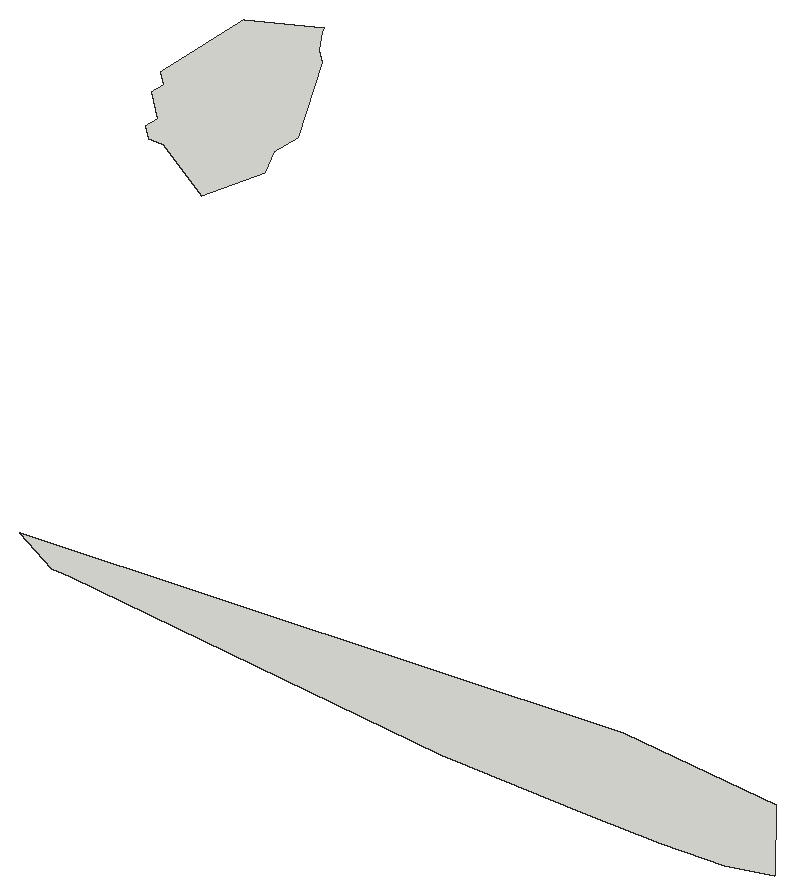
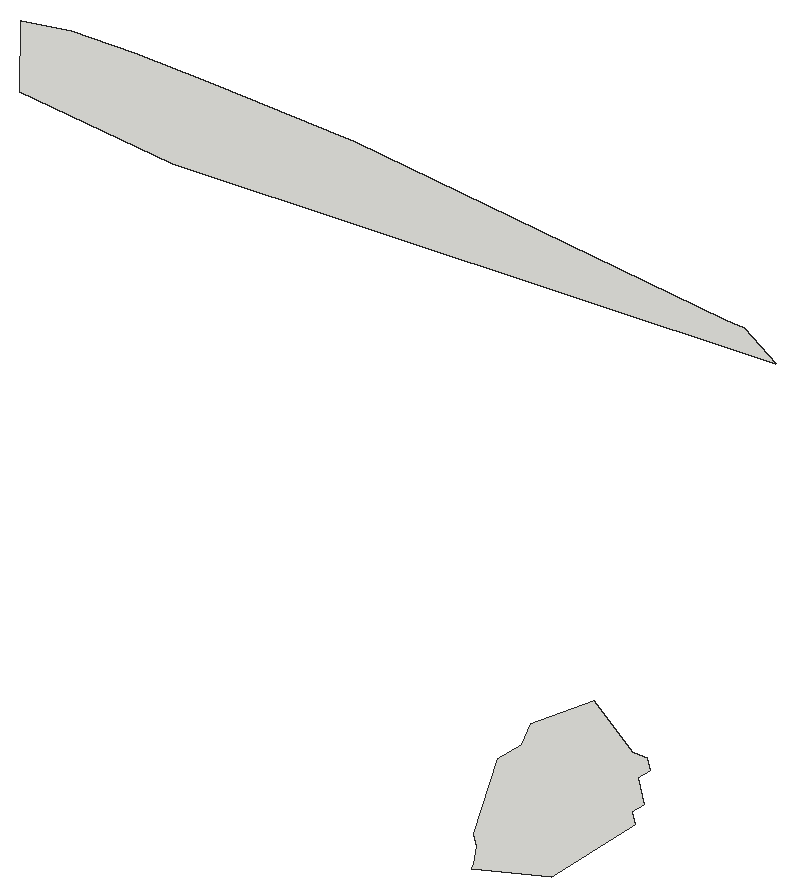
# SketchUp Ruby script. Lengths in inches.
U = 1.inch
M = Sketchup.active_model
def pt(a) = Geom::Point3d.new(a.map { |v| v * U })
def face(e, loops, mat)
  f = e.add_face(loops[0].map { |a| pt(a) })
  loops[1..].each { |l| e.add_face(l.map { |a| pt(a) }).erase! }
  f.material = f.back_material = mat if mat
  f
end
# faces: each face lists its corners as indices into pts; further lists are holes
def faces(e, pts, list, mat = nil) = list.each { |f| face(e, (f[0].is_a?(Array) ? f : [f]).map { |l| l.map { |i| pts[i] } }, mat) }
# xy, xz, yz: faces in a plane at the given z, y or x. An outline is a flat list of corners, or four numbers for a rectangle; further outlines are holes
def ring(l) = l.size == 4 ? [[l[0], l[1]], [l[2], l[1]], [l[2], l[3]], [l[0], l[3]]] : l.each_slice(2).to_a
def flat(e, list, mat, &to3) = list.each { |f| face(e, (f[0].is_a?(Array) ? f : [f]).map { |l| ring(l).map { |u, v| to3.(u, v) } }, mat) }
def xy(e, z, list, mat = nil) = flat(e, list, mat) { |x, y| [x, y, z] }
def xz(e, y, list, mat = nil) = flat(e, list, mat) { |x, z| [x, y, z] }
def yz(e, x, list, mat = nil) = flat(e, list, mat) { |y, z| [x, y, z] }
def lines(e, pts, list) = list.each { |a, b| e.add_line(pt(pts[a]), pt(pts[b])) }
# prism: a flat outline (further loops are holes) pulled along v
def prism(e, loops, v, mat = nil)
  f = face(e, loops, mat); d = Geom::Vector3d.new(v.map { |x| x * U })
  f.pushpull(f.normal.samedirection?(d) ? d.length : -d.length)
end
def box(e, o, s, mat = nil) = prism(e, [[o, [o[0] + s[0], o[1], o[2]], [o[0] + s[0], o[1] + s[1], o[2]], [o[0], o[1] + s[1], o[2]]]], [0, 0, s[2]], mat)
def at(x, y, z, deg = 0) = Geom::Transformation.translation(pt([x, y, z])) * Geom::Transformation.rotation(ORIGIN, Z_AXIS, deg.degrees)
def axes(o, x, y, z) = Geom::Transformation.new([*x, 0, *y, 0, *z, 0, *pt(o).to_a, 1])
def part(name) = M.definitions.add(name)
# library, detail: a bought-in or finely detailed component or shape, given as its bounding box
def library(name, o, s) = part(name).tap { |d| box(d.entities, o, s) }
def detail(e, o, s) = box(e.add_group.entities, o, s)
def put(e, d, t, mat = nil) = e.add_instance(d, t).tap { |i| i.material = mat if mat }
def group(e, t, mat = nil) = e.add_group.tap { |g| g.transformation = t; g.material = mat if mat }.entities
root = M.entities
xy(root,0,[[17.074,358.307,17.116,358.308,17.158,358.311,17.189,358.316,17.22,358.323,17.221,358.323,17.222,358.324,17.223,358.324,17.225,358.325,17.226,358.326,17.227,358.326,17.231,358.33,17.231,358.331,17.232,358.333,17.233,358.334,17.233,358.335,17.234,358.336,17.234,358.338,17.235,358.339,17.235,358.347,17.234,358.349,17.234,358.35,17.233,358.352,17.233,358.353,17.231,358.355,17.23,358.357,17.225,358.362,17.224,358.362,17.222,358.363,17.221,358.364,17.218,358.364,17.138,358.381,17.031,358.391,16.904,358.393,16.66,358.387,16.659,358.387,16.657,358.386,16.655,358.386,16.653,358.384,16.651,358.383,16.65,358.381,16.649,358.38,16.649,358.378,16.648,358.377,16.648,358.372,16.649,358.37,16.649,358.369,16.65,358.367,16.651,358.366,16.654,358.362,16.658,358.359,16.661,358.356,16.665,358.354,16.669,358.351,16.673,358.349,16.678,358.347,16.682,358.346,16.686,358.344,16.691,358.343,16.696,358.343,16.974,358.313],[16.493,358.704,16.495,358.704,16.497,358.705,16.498,358.705,16.502,358.707,16.503,358.708,16.504,358.71,16.505,358.711,16.507,358.715,16.508,358.718,16.508,358.721,16.509,358.723,16.509,358.735,16.508,358.737,16.503,358.758,16.496,358.778,16.462,358.852,16.46,358.856,16.457,358.86,16.455,358.863,16.452,358.867,16.449,358.87,16.445,358.873,16.442,358.875,16.438,358.878,16.43,358.882,16.429,358.882,16.428,358.883,16.42,358.883,16.419,358.882,16.416,358.882,16.416,358.881,16.415,358.88,16.414,358.88,16.412,358.878,16.411,358.878,16.411,358.877,16.409,358.875,16.409,358.874,16.408,358.873,16.408,358.872,16.404,358.859,16.4,358.833,16.4,358.815,16.402,358.803,16.403,358.798,16.405,358.792,16.409,358.782,16.414,358.771,16.42,358.762,16.434,358.742,16.442,358.733,16.45,358.726,16.459,358.719,16.469,358.712,16.472,358.71,16.476,358.708,16.488,358.705]])
